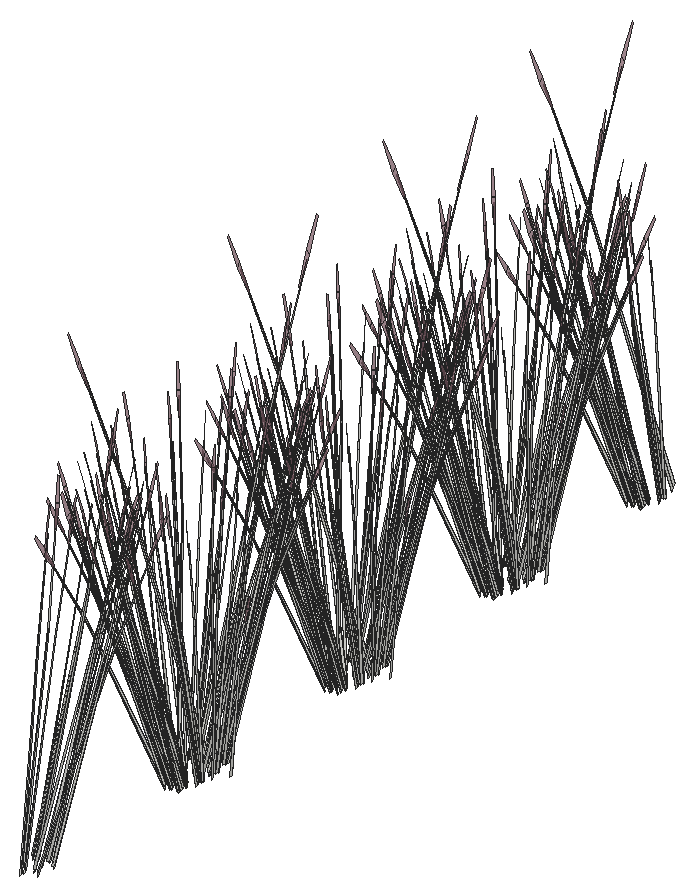
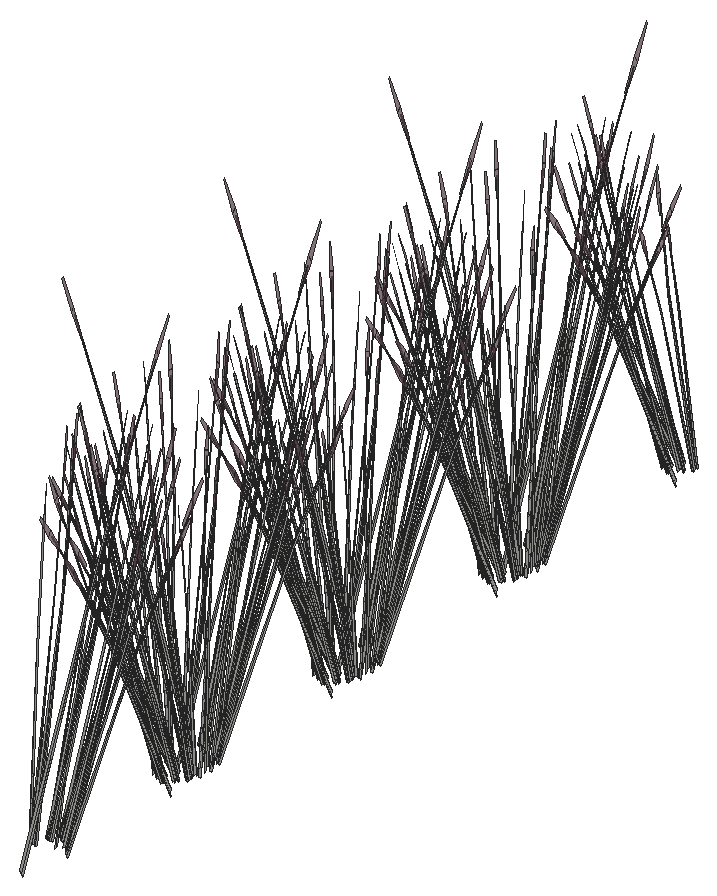
# SketchUp Ruby script. Lengths in inches.
U = 1.inch
M = Sketchup.active_model
def pt(a) = Geom::Point3d.new(a.map { |v| v * U })
def face(e, loops, mat)
  f = e.add_face(loops[0].map { |a| pt(a) })
  loops[1..].each { |l| e.add_face(l.map { |a| pt(a) }).erase! }
  f.material = f.back_material = mat if mat
  f
end
# faces: each face lists its corners as indices into pts; further lists are holes
def faces(e, pts, list, mat = nil) = list.each { |f| face(e, (f[0].is_a?(Array) ? f : [f]).map { |l| l.map { |i| pts[i] } }, mat) }
# xy, xz, yz: faces in a plane at the given z, y or x. An outline is a flat list of corners, or four numbers for a rectangle; further outlines are holes
def ring(l) = l.size == 4 ? [[l[0], l[1]], [l[2], l[1]], [l[2], l[3]], [l[0], l[3]]] : l.each_slice(2).to_a
def flat(e, list, mat, &to3) = list.each { |f| face(e, (f[0].is_a?(Array) ? f : [f]).map { |l| ring(l).map { |u, v| to3.(u, v) } }, mat) }
def xy(e, z, list, mat = nil) = flat(e, list, mat) { |x, y| [x, y, z] }
def xz(e, y, list, mat = nil) = flat(e, list, mat) { |x, z| [x, y, z] }
def yz(e, x, list, mat = nil) = flat(e, list, mat) { |y, z| [x, y, z] }
def lines(e, pts, list) = list.each { |a, b| e.add_line(pt(pts[a]), pt(pts[b])) }
# prism: a flat outline (further loops are holes) pulled along v
def prism(e, loops, v, mat = nil)
  f = face(e, loops, mat); d = Geom::Vector3d.new(v.map { |x| x * U })
  f.pushpull(f.normal.samedirection?(d) ? d.length : -d.length)
end
def box(e, o, s, mat = nil) = prism(e, [[o, [o[0] + s[0], o[1], o[2]], [o[0] + s[0], o[1] + s[1], o[2]], [o[0], o[1] + s[1], o[2]]]], [0, 0, s[2]], mat)
def at(x, y, z, deg = 0) = Geom::Transformation.translation(pt([x, y, z])) * Geom::Transformation.rotation(ORIGIN, Z_AXIS, deg.degrees)
def axes(o, x, y, z) = Geom::Transformation.new([*x, 0, *y, 0, *z, 0, *pt(o).to_a, 1])
def part(name) = M.definitions.add(name)
# library, detail: a bought-in or finely detailed component or shape, given as its bounding box
def library(name, o, s) = part(name).tap { |d| box(d.entities, o, s) }
def detail(e, o, s) = box(e.add_group.entities, o, s)
def put(e, d, t, mat = nil) = e.add_instance(d, t).tap { |i| i.material = mat if mat }
def group(e, t, mat = nil) = e.add_group.tap { |g| g.transformation = t; g.material = mat if mat }.entities
root = M.entities
M.materials.add("LightPink_Translucent").color = [144, 107, 117]
M.materials["LightPink_Translucent"].alpha = 0.75
c1 = part("blade")
p = [[2.15,0.21,22],[0,0.17,0],[0.09,0.45,0],[2.18,0.31,22],[2.29,0.31,22],[0.38,0.45,0],
  [2.48,0.24,33],[2.49,0.24,33],[2.48,0.22,33]]
faces(c1.entities,p,[[0,1,2,3],[4,5,2,3],[6,3,4,7],[8,0,3,6]])
c2 = part("seeds")
p = [[0.3,-0.1,1.38],[-0.01,-0.03,1.59],[-0.01,-0.03,0.03],[0.14,-0.07,-0.07],[0.29,-0.03,3],[0.15,0.01,3.11]]
faces(c2.entities,p,[[0,1,2,3],[1,0,4,5]],"LightPink_Translucent")
c3 = part("blade with seeds")
put(c3.entities,c1,at(0,0,0))
put(c3.entities,c2,axes([2.4,0.25,30.99],[1.5799,-0.05474,1.17369],[-0.12525,1.92788,0.29478],[-0.07173,-0.02425,1.56792]))
put(root,c3,axes([251.98,134.81,2.85],[0.15252,-0.52338,-0.08826],[0.22088,0.30152,-0.48986],[0.07678,0.14787,0.74434]))
put(root,c3,axes([250.875,132.91,2.01],[0.06393,-0.18788,1.24382],[0.16142,0.50711,0.10057],[-0.11071,0.23094,0.53172]))
put(root,c3,axes([250.67,133.46,2.59],[0.06575,0.55831,-0.37087],[-0.24901,0.09767,-0.28727],[-0.07136,0.14996,0.70962]))
put(root,c3,axes([252.16,134.55,2.59],[0.25257,-0.14535,-0.37087],[0.04418,0.55045,-0.28727],[0.06784,0.15774,0.70962]))
put(root,c3,axes([250.83,133.375,2.01],[0.04766,-0.21017,1.24382],[0.19993,0.43493,0.10057],[-0.09019,0.27107,0.53172]))
put(root,c3,axes([250.88,134.56,2.48],[-0.17318,0.32193,-0.25703],[-0.16394,-0.36759,0.33183],[-0.02494,0.18677,0.63492]))
put(root,c3,axes([251.38,134.83,2.85],[0.25047,-0.28468,-0.08826],[0.12309,0.50526,-0.48986],[0.03305,0.21292,0.74434]))
put(root,c3,axes([251.06,134.41,2.83],[0.18323,0.41084,-0.41166],[-0.19356,0.3598,-0.31887],[-0.02788,0.20874,0.78768]))
put(root,c3,axes([251.6,134.81,2.59],[0.25161,0.15328,-0.37087],[-0.08624,0.52553,-0.28727],[0.02307,0.21159,0.70962]))
put(root,c3,axes([251.74,133.72,2.01],[-0.05851,-0.19632,1.24382],[0.27036,-0.16528,0.10057],[0.0611,0.3082,0.53172]))
put(root,c3,axes([251.48,135.13,2.48],[-0.07716,0.47021,-0.25703],[-0.22512,-0.13715,0.33183],[0.02064,0.18932,0.63492]))
put(root,c3,axes([251,134.22,3.07],[-0.00666,0.56559,-0.57235],[-0.28045,-0.03799,0.06907],[-0.0296,0.23961,0.80965]))
put(root,c3,axes([251.26,133.82,2.01],[-0.00626,-0.23468,1.24382],[0.27152,0.15569,0.10057],[-0.01679,0.33444,0.53172]))
put(root,c3,axes([251.51,134.71,2.81],[0.12216,0.49718,-0.51563],[-0.25147,0.27708,0.06223],[0.02857,0.24022,0.72942]))
put(root,c3,axes([250.9,135.02,1.63],[0.00562,-0.31565,1.12021],[0.25293,0.16673,0.1548],[-0.02192,0.33641,0.52896]))
put(root,c3,axes([251.1,147.52,2.01],[0.05851,0.19632,1.24382],[-0.27036,0.16528,0.10057],[-0.0611,-0.3082,0.53172]))
put(root,c3,axes([251.82,147.67,2.81],[-0.12216,-0.49718,-0.51563],[0.25147,-0.27708,0.06223],[-0.02857,-0.24022,0.72942]))
put(root,c3,axes([252.33,148.15,2.81],[0.00666,-0.56559,-0.51563],[0.28045,0.03799,0.06223],[0.0296,-0.23961,0.72942]))
put(root,c3,axes([251.84,147.24,2.48],[0.07716,-0.47021,-0.25703],[0.22512,0.13715,0.33183],[-0.02064,-0.18932,0.63492]))
put(root,c3,axes([252.01,147.87,2.01],[-0.04766,0.21017,1.24382],[-0.19993,-0.43493,0.10057],[0.09019,-0.27107,0.53172]))
put(root,c3,axes([251.73,147.57,2.59],[-0.25161,-0.15328,-0.37087],[0.08624,-0.52553,-0.28727],[-0.02307,-0.21159,0.70962]))
put(root,c3,axes([252.27,147.97,2.59],[-0.18323,-0.41084,-0.37087],[0.19356,-0.3598,-0.28727],[0.02788,-0.20874,0.70962]))
put(root,c3,axes([251.94,147.54,2.85],[-0.25047,0.28468,-0.08826],[-0.12309,-0.50526,-0.48986],[-0.03305,-0.21292,0.74434]))
put(root,c3,axes([252.46,148.18,2.85],[-0.2813,-0.0303,-0.08826],[0.00769,-0.57361,-0.48986],[0.01954,-0.22092,0.74434]))
put(root,c3,axes([252.44,147.8125,2.48],[0.17318,-0.32193,-0.25703],[0.16394,0.36759,0.33183],[0.02494,-0.18677,0.63492]))
put(root,c3,axes([251.27,147.81,2.81],[-0.21825,-0.29555,-0.51563],[0.15511,-0.5179,0.06223],[-0.07907,-0.17646,0.72942]))
put(root,c3,axes([251.19,147.42,2.48],[-0.03953,-0.49251,-0.25703],[0.22598,-0.13005,0.33183],[-0.0607,-0.14114,0.63492]))
put(root,c3,axes([250.71,148.13,2.01],[0.09507,0.10535,1.24382],[-0.19675,0.44195,0.10057],[-0.12263,-0.19937,0.53172]))
put(root,c3,axes([251.17,147.82,2.59],[-0.25257,0.14535,-0.37087],[-0.04418,-0.55045,-0.28727],[-0.06784,-0.15774,0.70962]))
put(root,c3,axes([252.66,149.14,2.81],[0.1337,-0.48245,-0.51563],[0.23429,0.34287,0.06223],[0.07983,-0.1748,0.72942]))
put(root,c3,axes([252.65,148.91,2.59],[-0.06575,-0.55831,-0.37087],[0.24901,-0.09767,-0.28727],[0.07136,-0.14996,0.70962]))
put(root,c3,axes([252.77,149.31,2.85],[-0.23676,-0.33715,-0.08826],[0.1364,-0.48826,-0.48986],[0.06689,-0.16972,0.74434]))
put(root,c3,axes([251.79,151.15,1.61],[0.22119,0.24656,1.09782],[-0.21669,0.53118,0.43413],[-0.09706,-0.31482,0.92034]))
put(root,c3,axes([252.84,148.97,2.48],[0.2228,-0.08739,-0.25703],[0.05883,0.49954,0.33183],[0.06385,-0.13418,0.63492]))
put(root,c3,axes([250.67,148.28,2.48],[-0.14563,-0.38283,-0.25703],[0.16629,-0.3624,0.33183],[-0.08449,-0.05514,0.63492]))
put(root,c3,axes([250.82,148.54,2.81],[-0.25586,-0.01472,-0.51563],[0.01718,-0.61995,0.06223],[-0.1084,-0.06542,0.72942]))
put(root,c3,axes([250.74,148.66,2.59],[-0.18586,0.40503,-0.37087],[-0.16277,-0.42787,-0.28727],[-0.09443,-0.06163,0.70962]))
put(root,c3,axes([250.84,148.24,2.85],[-0.0137,0.62183,-0.08826],[-0.25949,-0.017,-0.48986],[-0.09994,-0.0432,0.74434]))
put(root,c3,axes([252.78,150.625,2.85],[-0.12878,-0.55367,-0.08826],[0.22857,-0.27208,-0.48986],[0.09632,-0.07305,0.74434]))
put(root,c3,axes([252.77,150.15,2.59],[0.06934,-0.55619,-0.37087],[0.23774,0.19064,-0.28727],[0.09572,-0.051,0.70962]))
put(root,c3,axes([250.51,149.1,2.01],[0.10617,-0.01385,1.24382],[-0.07043,0.60021,0.10057],[-0.1513,-0.03712,0.53172]))
put(root,c3,axes([252.72,150.35,2.81],[0.22491,-0.27005,-0.51563],[0.12534,0.55588,0.06223],[0.10867,-0.06315,0.72942]))
put(root,c3,axes([252.91,150.4,2.48],[0.21272,0.17057,-0.25703],[-0.06204,0.49764,0.33183],[0.08564,-0.04563,0.63492]))
put(root,c3,axes([250.41,149.61,2.48],[-0.21272,-0.17057,-0.25703],[0.06204,-0.49764,0.33183],[-0.08564,0.04563,0.63492]))
put(root,c3,axes([252.33,149.79,2.01],[-0.10617,0.01385,1.24382],[0.07043,-0.60021,0.10057],[0.1513,0.03712,0.53172]))
put(root,c3,axes([251.0625,149.53,1.62],[0.07276,-0.08845,1.2851],[0.02509,0.61759,0.10057],[-0.15759,0.08195,0.4593]))
put(root,c3,axes([250.56,149.87,2.59],[-0.06934,0.55619,-0.37087],[-0.23774,-0.19064,-0.28727],[-0.09572,0.051,0.70962]))
put(root,c3,axes([250.55,149.39,2.85],[0.12878,0.55367,-0.08826],[-0.22857,0.27208,-0.48986],[-0.09632,0.07305,0.74434]))
put(root,c3,axes([253.09,151.79,2.04],[-0.04899,-0.514,-0.02534],[0.23154,-0.11817,-0.1149],[0.04835,0.03259,0.37899]))
put(root,c3,axes([252.49,151.78,2.85],[0.0137,-0.62183,-0.08826],[0.25949,0.017,-0.48986],[0.09994,0.0432,0.74434]))
put(root,c3,axes([250.55,150.15,2.01],[0.08881,-0.12933,1.24382],[0.07477,0.59764,0.10057],[-0.13942,0.13507,0.53172]))
put(root,c3,axes([252.5,151.48,2.81],[0.25586,0.01472,-0.51563],[-0.01718,0.61995,0.06223],[0.1084,0.06542,0.72942]))
put(root,c3,axes([252.66,151.73,2.48],[0.14563,0.38283,-0.25703],[-0.16629,0.3624,0.33183],[0.08449,0.05514,0.63492]))
put(root,c3,axes([250.49,151.05,2.48],[-0.2228,0.08739,-0.25703],[-0.05883,-0.49954,0.33183],[-0.06385,0.13418,0.63492]))
put(root,c3,axes([252.13,150.75,2.01],[-0.09507,-0.10535,1.24382],[0.19675,-0.44195,0.10057],[0.12263,0.19937,0.53172]))
put(root,c3,axes([252.15,149.36,2.44],[-0.22117,-0.3177,1.00363],[0.23354,-0.49464,0.43304],[0.07136,0.29809,0.97011]))
put(root,c3,axes([250.56,150.71,2.85],[0.23676,0.33715,-0.08826],[-0.1364,0.48826,-0.48986],[-0.06689,0.16972,0.74434]))
put(root,c3,axes([251.98,152.45,2.85],[0.15252,-0.52338,-0.08826],[0.22088,0.30152,-0.48986],[0.07678,0.14787,0.74434]))
put(root,c3,axes([250.875,150.55,2.01],[0.06393,-0.18788,1.24382],[0.16142,0.50711,0.10057],[-0.11071,0.23094,0.53172]))
put(root,c3,axes([250.67,151.11,2.59],[0.06575,0.55831,-0.37087],[-0.24901,0.09767,-0.28727],[-0.07136,0.14996,0.70962]))
put(root,c3,axes([252.16,152.19,2.59],[0.25257,-0.14535,-0.37087],[0.04418,0.55045,-0.28727],[0.06784,0.15774,0.70962]))
put(root,c3,axes([250.83,151.02,2.01],[0.04766,-0.21017,1.24382],[0.19993,0.43493,0.10057],[-0.09019,0.27107,0.53172]))
put(root,c3,axes([250.88,152.2,2.48],[-0.17318,0.32193,-0.25703],[-0.16394,-0.36759,0.33183],[-0.02494,0.18677,0.63492]))
put(root,c3,axes([251.38,152.47,2.85],[0.25047,-0.28468,-0.08826],[0.12309,0.50526,-0.48986],[0.03305,0.21292,0.74434]))
put(root,c3,axes([251.06,152.05,2.83],[0.18323,0.41084,-0.41166],[-0.19356,0.3598,-0.31887],[-0.02788,0.20874,0.78768]))
put(root,c3,axes([251.6,152.45,2.59],[0.25161,0.15328,-0.37087],[-0.08624,0.52553,-0.28727],[0.02307,0.21159,0.70962]))
put(root,c3,axes([251.74,151.36,2.01],[-0.05851,-0.19632,1.24382],[0.27036,-0.16528,0.10057],[0.0611,0.3082,0.53172]))
put(root,c3,axes([251.48,152.77,2.48],[-0.07716,0.47021,-0.25703],[-0.22512,-0.13715,0.33183],[0.02064,0.18932,0.63492]))
put(root,c3,axes([251,151.86,3.07],[-0.00666,0.56559,-0.57235],[-0.28045,-0.03799,0.06907],[-0.0296,0.23961,0.80965]))
put(root,c3,axes([251.26,151.46,2.01],[-0.00626,-0.23468,1.24382],[0.27152,0.15569,0.10057],[-0.01679,0.33444,0.53172]))
put(root,c3,axes([251.51,152.35,2.81],[0.12216,0.49718,-0.51563],[-0.25147,0.27708,0.06223],[0.02857,0.24022,0.72942]))
put(root,c3,axes([250.9,152.66,1.63],[0.00562,-0.31565,1.12021],[0.25293,0.16673,0.1548],[-0.02192,0.33641,0.52896]))
put(root,c3,axes([251.1,163.79,2.01],[0.05851,0.19632,1.24382],[-0.27036,0.16528,0.10057],[-0.0611,-0.3082,0.53172]))
put(root,c3,axes([251.82,163.9375,2.81],[-0.12216,-0.49718,-0.51563],[0.25147,-0.27708,0.06223],[-0.02857,-0.24022,0.72942]))
put(root,c3,axes([252.33,164.42,2.81],[0.00666,-0.56559,-0.51563],[0.28045,0.03799,0.06223],[0.0296,-0.23961,0.72942]))
put(root,c3,axes([251.84,163.51,2.48],[0.07716,-0.47021,-0.25703],[0.22512,0.13715,0.33183],[-0.02064,-0.18932,0.63492]))
put(root,c3,axes([252.01,164.14,2.01],[-0.04766,0.21017,1.24382],[-0.19993,-0.43493,0.10057],[0.09019,-0.27107,0.53172]))
put(root,c3,axes([251.73,163.84,2.59],[-0.25161,-0.15328,-0.37087],[0.08624,-0.52553,-0.28727],[-0.02307,-0.21159,0.70962]))
put(root,c3,axes([252.27,164.23,2.59],[-0.18323,-0.41084,-0.37087],[0.19356,-0.3598,-0.28727],[0.02788,-0.20874,0.70962]))
put(root,c3,axes([251.94,163.8125,2.85],[-0.25047,0.28468,-0.08826],[-0.12309,-0.50526,-0.48986],[-0.03305,-0.21292,0.74434]))
put(root,c3,axes([252.46,164.45,2.85],[-0.2813,-0.0303,-0.08826],[0.00769,-0.57361,-0.48986],[0.01954,-0.22092,0.74434]))
put(root,c3,axes([252.44,164.08,2.48],[0.17318,-0.32193,-0.25703],[0.16394,0.36759,0.33183],[0.02494,-0.18677,0.63492]))
put(root,c3,axes([251.27,164.08,2.81],[-0.21825,-0.29555,-0.51563],[0.15511,-0.5179,0.06223],[-0.07907,-0.17646,0.72942]))
put(root,c3,axes([251.19,163.6875,2.48],[-0.03953,-0.49251,-0.25703],[0.22598,-0.13005,0.33183],[-0.0607,-0.14114,0.63492]))
put(root,c3,axes([250.71,164.4,2.01],[0.09507,0.10535,1.24382],[-0.19675,0.44195,0.10057],[-0.12263,-0.19937,0.53172]))
put(root,c3,axes([251.17,164.09,2.59],[-0.25257,0.14535,-0.37087],[-0.04418,-0.55045,-0.28727],[-0.06784,-0.15774,0.70962]))
put(root,c3,axes([252.66,165.41,2.81],[0.1337,-0.48245,-0.51563],[0.23429,0.34287,0.06223],[0.07983,-0.1748,0.72942]))
put(root,c3,axes([252.65,165.18,2.59],[-0.06575,-0.55831,-0.37087],[0.24901,-0.09767,-0.28727],[0.07136,-0.14996,0.70962]))
put(root,c3,axes([252.77,165.58,2.85],[-0.23676,-0.33715,-0.08826],[0.1364,-0.48826,-0.48986],[0.06689,-0.16972,0.74434]))
put(root,c3,axes([251.79,167.42,1.61],[0.22119,0.24656,1.09782],[-0.21669,0.53118,0.43413],[-0.09706,-0.31482,0.92034]))
put(root,c3,axes([252.84,165.24,2.48],[0.2228,-0.08739,-0.25703],[0.05883,0.49954,0.33183],[0.06385,-0.13418,0.63492]))
put(root,c3,axes([250.67,164.55,2.48],[-0.14563,-0.38283,-0.25703],[0.16629,-0.3624,0.33183],[-0.08449,-0.05514,0.63492]))
put(root,c3,axes([250.82,164.81,2.81],[-0.25586,-0.01472,-0.51563],[0.01718,-0.61995,0.06223],[-0.1084,-0.06542,0.72942]))
put(root,c3,axes([250.74,164.93,2.59],[-0.18586,0.40503,-0.37087],[-0.16277,-0.42787,-0.28727],[-0.09443,-0.06163,0.70962]))
put(root,c3,axes([250.84,164.51,2.85],[-0.0137,0.62183,-0.08826],[-0.25949,-0.017,-0.48986],[-0.09994,-0.0432,0.74434]))
put(root,c3,axes([252.78,166.9,2.85],[-0.12878,-0.55367,-0.08826],[0.22857,-0.27208,-0.48986],[0.09632,-0.07305,0.74434]))
put(root,c3,axes([252.77,166.42,2.59],[0.06934,-0.55619,-0.37087],[0.23774,0.19064,-0.28727],[0.09572,-0.051,0.70962]))
put(root,c3,axes([250.51,165.37,2.01],[0.10617,-0.01385,1.24382],[-0.07043,0.60021,0.10057],[-0.1513,-0.03712,0.53172]))
put(root,c3,axes([252.72,166.62,2.81],[0.22491,-0.27005,-0.51563],[0.12534,0.55588,0.06223],[0.10867,-0.06315,0.72942]))
put(root,c3,axes([252.91,166.67,2.48],[0.21272,0.17057,-0.25703],[-0.06204,0.49764,0.33183],[0.08564,-0.04563,0.63492]))
put(root,c3,axes([250.41,165.88,2.48],[-0.21272,-0.17057,-0.25703],[0.06204,-0.49764,0.33183],[-0.08564,0.04563,0.63492]))
put(root,c3,axes([252.33,166.06,2.01],[-0.10617,0.01385,1.24382],[0.07043,-0.60021,0.10057],[0.1513,0.03712,0.53172]))
put(root,c3,axes([251.0625,165.8,1.62],[0.07276,-0.08845,1.2851],[0.02509,0.61759,0.10057],[-0.15759,0.08195,0.4593]))
put(root,c3,axes([250.56,166.13,2.59],[-0.06934,0.55619,-0.37087],[-0.23774,-0.19064,-0.28727],[-0.09572,0.051,0.70962]))
put(root,c3,axes([250.55,165.66,2.85],[0.12878,0.55367,-0.08826],[-0.22857,0.27208,-0.48986],[-0.09632,0.07305,0.74434]))
put(root,c3,axes([253.09,168.0625,2.04],[-0.04899,-0.514,-0.02534],[0.23154,-0.11817,-0.1149],[0.04835,0.03259,0.37899]))
put(root,c3,axes([252.49,168.05,2.85],[0.0137,-0.62183,-0.08826],[0.25949,0.017,-0.48986],[0.09994,0.0432,0.74434]))
put(root,c3,axes([250.55,166.42,2.01],[0.08881,-0.12933,1.24382],[0.07477,0.59764,0.10057],[-0.13942,0.13507,0.53172]))
put(root,c3,axes([252.5,167.75,2.81],[0.25586,0.01472,-0.51563],[-0.01718,0.61995,0.06223],[0.1084,0.06542,0.72942]))
put(root,c3,axes([252.66,168,2.48],[0.14563,0.38283,-0.25703],[-0.16629,0.3624,0.33183],[0.08449,0.05514,0.63492]))
put(root,c3,axes([250.49,167.32,2.48],[-0.2228,0.08739,-0.25703],[-0.05883,-0.49954,0.33183],[-0.06385,0.13418,0.63492]))
put(root,c3,axes([252.13,167.02,2.01],[-0.09507,-0.10535,1.24382],[0.19675,-0.44195,0.10057],[0.12263,0.19937,0.53172]))
put(root,c3,axes([252.15,165.63,2.44],[-0.22117,-0.3177,1.00363],[0.23354,-0.49464,0.43304],[0.07136,0.29809,0.97011]))
put(root,c3,axes([250.56,166.98,2.85],[0.23676,0.33715,-0.08826],[-0.1364,0.48826,-0.48986],[-0.06689,0.16972,0.74434]))
put(root,c3,axes([251.98,168.72,2.85],[0.15252,-0.52338,-0.08826],[0.22088,0.30152,-0.48986],[0.07678,0.14787,0.74434]))
put(root,c3,axes([250.875,166.82,2.01],[0.06393,-0.18788,1.24382],[0.16142,0.50711,0.10057],[-0.11071,0.23094,0.53172]))
put(root,c3,axes([250.67,167.375,2.59],[0.06575,0.55831,-0.37087],[-0.24901,0.09767,-0.28727],[-0.07136,0.14996,0.70962]))
put(root,c3,axes([252.16,168.46,2.59],[0.25257,-0.14535,-0.37087],[0.04418,0.55045,-0.28727],[0.06784,0.15774,0.70962]))
put(root,c3,axes([250.83,167.29,2.01],[0.04766,-0.21017,1.24382],[0.19993,0.43493,0.10057],[-0.09019,0.27107,0.53172]))
put(root,c3,axes([250.88,168.47,2.48],[-0.17318,0.32193,-0.25703],[-0.16394,-0.36759,0.33183],[-0.02494,0.18677,0.63492]))
put(root,c3,axes([251.38,168.74,2.85],[0.25047,-0.28468,-0.08826],[0.12309,0.50526,-0.48986],[0.03305,0.21292,0.74434]))
put(root,c3,axes([251.06,168.32,2.83],[0.18323,0.41084,-0.41166],[-0.19356,0.3598,-0.31887],[-0.02788,0.20874,0.78768]))
put(root,c3,axes([251.6,168.72,2.59],[0.25161,0.15328,-0.37087],[-0.08624,0.52553,-0.28727],[0.02307,0.21159,0.70962]))
put(root,c3,axes([251.74,167.63,2.01],[-0.05851,-0.19632,1.24382],[0.27036,-0.16528,0.10057],[0.0611,0.3082,0.53172]))
put(root,c3,axes([251.48,169.04,2.48],[-0.07716,0.47021,-0.25703],[-0.22512,-0.13715,0.33183],[0.02064,0.18932,0.63492]))
put(root,c3,axes([251,168.13,3.07],[-0.00666,0.56559,-0.57235],[-0.28045,-0.03799,0.06907],[-0.0296,0.23961,0.80965]))
put(root,c3,axes([251.26,167.73,2.01],[-0.00626,-0.23468,1.24382],[0.27152,0.15569,0.10057],[-0.01679,0.33444,0.53172]))
put(root,c3,axes([251.51,168.62,2.81],[0.12216,0.49718,-0.51563],[-0.25147,0.27708,0.06223],[0.02857,0.24022,0.72942]))
put(root,c3,axes([251.1,179.64,2.01],[0.05851,0.19632,1.24382],[-0.27036,0.16528,0.10057],[-0.0611,-0.3082,0.53172]))
put(root,c3,axes([250.9,168.93,1.63],[0.00562,-0.31565,1.12021],[0.25293,0.16673,0.1548],[-0.02192,0.33641,0.52896]))
put(root,c3,axes([251.82,179.79,2.81],[-0.12216,-0.49718,-0.51563],[0.25147,-0.27708,0.06223],[-0.02857,-0.24022,0.72942]))
put(root,c3,axes([252.33,180.27,2.81],[0.00666,-0.56559,-0.51563],[0.28045,0.03799,0.06223],[0.0296,-0.23961,0.72942]))
put(root,c3,axes([251.84,179.37,2.48],[0.07716,-0.47021,-0.25703],[0.22512,0.13715,0.33183],[-0.02064,-0.18932,0.63492]))
put(root,c3,axes([252.01,179.99,2.01],[-0.04766,0.21017,1.24382],[-0.19993,-0.43493,0.10057],[0.09019,-0.27107,0.53172]))
put(root,c3,axes([251.73,179.6875,2.59],[-0.25161,-0.15328,-0.37087],[0.08624,-0.52553,-0.28727],[-0.02307,-0.21159,0.70962]))
put(root,c3,axes([252.27,180.09,2.59],[-0.18323,-0.41084,-0.37087],[0.19356,-0.3598,-0.28727],[0.02788,-0.20874,0.70962]))
put(root,c3,axes([251.94,179.66,2.85],[-0.25047,0.28468,-0.08826],[-0.12309,-0.50526,-0.48986],[-0.03305,-0.21292,0.74434]))
put(root,c3,axes([252.46,180.3,2.85],[-0.2813,-0.0303,-0.08826],[0.00769,-0.57361,-0.48986],[0.01954,-0.22092,0.74434]))
put(root,c3,axes([252.44,179.93,2.48],[0.17318,-0.32193,-0.25703],[0.16394,0.36759,0.33183],[0.02494,-0.18677,0.63492]))
put(root,c3,axes([251.27,179.93,2.81],[-0.21825,-0.29555,-0.51563],[0.15511,-0.5179,0.06223],[-0.07907,-0.17646,0.72942]))
put(root,c3,axes([251.19,179.54,2.48],[-0.03953,-0.49251,-0.25703],[0.22598,-0.13005,0.33183],[-0.0607,-0.14114,0.63492]))
put(root,c3,axes([250.71,180.25,2.01],[0.09507,0.10535,1.24382],[-0.19675,0.44195,0.10057],[-0.12263,-0.19937,0.53172]))
put(root,c3,axes([251.17,179.94,2.59],[-0.25257,0.14535,-0.37087],[-0.04418,-0.55045,-0.28727],[-0.06784,-0.15774,0.70962]))
put(root,c3,axes([252.66,181.26,2.81],[0.1337,-0.48245,-0.51563],[0.23429,0.34287,0.06223],[0.07983,-0.1748,0.72942]))
put(root,c3,axes([252.65,181.03,2.59],[-0.06575,-0.55831,-0.37087],[0.24901,-0.09767,-0.28727],[0.07136,-0.14996,0.70962]))
put(root,c3,axes([252.77,181.43,2.85],[-0.23676,-0.33715,-0.08826],[0.1364,-0.48826,-0.48986],[0.06689,-0.16972,0.74434]))
put(root,c3,axes([251.79,183.27,1.61],[0.22119,0.24656,1.09782],[-0.21669,0.53118,0.43413],[-0.09706,-0.31482,0.92034]))
put(root,c3,axes([252.84,181.09,2.48],[0.2228,-0.08739,-0.25703],[0.05883,0.49954,0.33183],[0.06385,-0.13418,0.63492]))
put(root,c3,axes([250.67,180.4,2.48],[-0.14563,-0.38283,-0.25703],[0.16629,-0.3624,0.33183],[-0.08449,-0.05514,0.63492]))
put(root,c3,axes([250.82,180.66,2.81],[-0.25586,-0.01472,-0.51563],[0.01718,-0.61995,0.06223],[-0.1084,-0.06542,0.72942]))
put(root,c3,axes([250.74,180.78,2.59],[-0.18586,0.40503,-0.37087],[-0.16277,-0.42787,-0.28727],[-0.09443,-0.06163,0.70962]))
put(root,c3,axes([250.84,180.36,2.85],[-0.0137,0.62183,-0.08826],[-0.25949,-0.017,-0.48986],[-0.09994,-0.0432,0.74434]))
put(root,c3,axes([252.78,182.75,2.85],[-0.12878,-0.55367,-0.08826],[0.22857,-0.27208,-0.48986],[0.09632,-0.07305,0.74434]))
put(root,c3,axes([252.77,182.27,2.59],[0.06934,-0.55619,-0.37087],[0.23774,0.19064,-0.28727],[0.09572,-0.051,0.70962]))
put(root,c3,axes([250.51,181.22,2.01],[0.10617,-0.01385,1.24382],[-0.07043,0.60021,0.10057],[-0.1513,-0.03712,0.53172]))
put(root,c3,axes([252.72,182.47,2.81],[0.22491,-0.27005,-0.51563],[0.12534,0.55588,0.06223],[0.10867,-0.06315,0.72942]))
put(root,c3,axes([252.91,182.53,2.48],[0.21272,0.17057,-0.25703],[-0.06204,0.49764,0.33183],[0.08564,-0.04563,0.63492]))
put(root,c3,axes([250.41,181.73,2.48],[-0.21272,-0.17057,-0.25703],[0.06204,-0.49764,0.33183],[-0.08564,0.04563,0.63492]))
put(root,c3,axes([252.33,181.91,2.01],[-0.10617,0.01385,1.24382],[0.07043,-0.60021,0.10057],[0.1513,0.03712,0.53172]))
put(root,c3,axes([251.0625,181.65,1.62],[0.07276,-0.08845,1.2851],[0.02509,0.61759,0.10057],[-0.15759,0.08195,0.4593]))
put(root,c3,axes([250.56,181.99,2.59],[-0.06934,0.55619,-0.37087],[-0.23774,-0.19064,-0.28727],[-0.09572,0.051,0.70962]))
put(root,c3,axes([250.55,181.51,2.85],[0.12878,0.55367,-0.08826],[-0.22857,0.27208,-0.48986],[-0.09632,0.07305,0.74434]))
put(root,c3,axes([253.09,183.91,2.04],[-0.04899,-0.514,-0.02534],[0.23154,-0.11817,-0.1149],[0.04835,0.03259,0.37899]))
put(root,c3,axes([252.49,183.9,2.85],[0.0137,-0.62183,-0.08826],[0.25949,0.017,-0.48986],[0.09994,0.0432,0.74434]))
put(root,c3,axes([250.55,182.27,2.01],[0.08881,-0.12933,1.24382],[0.07477,0.59764,0.10057],[-0.13942,0.13507,0.53172]))
put(root,c3,axes([252.5,183.6,2.81],[0.25586,0.01472,-0.51563],[-0.01718,0.61995,0.06223],[0.1084,0.06542,0.72942]))
put(root,c3,axes([252.66,183.85,2.48],[0.14563,0.38283,-0.25703],[-0.16629,0.3624,0.33183],[0.08449,0.05514,0.63492]))
put(root,c3,axes([250.49,183.17,2.48],[-0.2228,0.08739,-0.25703],[-0.05883,-0.49954,0.33183],[-0.06385,0.13418,0.63492]))
put(root,c3,axes([252.13,182.87,2.01],[-0.09507,-0.10535,1.24382],[0.19675,-0.44195,0.10057],[0.12263,0.19937,0.53172]))
put(root,c3,axes([252.15,181.49,2.44],[-0.22117,-0.3177,1.00363],[0.23354,-0.49464,0.43304],[0.07136,0.29809,0.97011]))
put(root,c3,axes([250.56,182.83,2.85],[0.23676,0.33715,-0.08826],[-0.1364,0.48826,-0.48986],[-0.06689,0.16972,0.74434]))
put(root,c3,axes([251.98,184.57,2.85],[0.15252,-0.52338,-0.08826],[0.22088,0.30152,-0.48986],[0.07678,0.14787,0.74434]))
put(root,c3,axes([250.875,182.68,2.01],[0.06393,-0.18788,1.24382],[0.16142,0.50711,0.10057],[-0.11071,0.23094,0.53172]))
put(root,c3,axes([250.67,183.23,2.59],[0.06575,0.55831,-0.37087],[-0.24901,0.09767,-0.28727],[-0.07136,0.14996,0.70962]))
put(root,c3,axes([252.16,184.3125,2.59],[0.25257,-0.14535,-0.37087],[0.04418,0.55045,-0.28727],[0.06784,0.15774,0.70962]))
put(root,c3,axes([250.83,183.14,2.01],[0.04766,-0.21017,1.24382],[0.19993,0.43493,0.10057],[-0.09019,0.27107,0.53172]))
put(root,c3,axes([250.88,184.32,2.48],[-0.17318,0.32193,-0.25703],[-0.16394,-0.36759,0.33183],[-0.02494,0.18677,0.63492]))
put(root,c3,axes([251.38,184.6,2.85],[0.25047,-0.28468,-0.08826],[0.12309,0.50526,-0.48986],[0.03305,0.21292,0.74434]))
put(root,c3,axes([251.06,184.17,2.83],[0.18323,0.41084,-0.41166],[-0.19356,0.3598,-0.31887],[-0.02788,0.20874,0.78768]))
put(root,c3,axes([251.6,184.57,2.59],[0.25161,0.15328,-0.37087],[-0.08624,0.52553,-0.28727],[0.02307,0.21159,0.70962]))
put(root,c3,axes([251.74,183.49,2.01],[-0.05851,-0.19632,1.24382],[0.27036,-0.16528,0.10057],[0.0611,0.3082,0.53172]))
put(root,c3,axes([251.48,184.89,2.48],[-0.07716,0.47021,-0.25703],[-0.22512,-0.13715,0.33183],[0.02064,0.18932,0.63492]))
put(root,c3,axes([251,183.98,3.07],[-0.00666,0.56559,-0.57235],[-0.28045,-0.03799,0.06907],[-0.0296,0.23961,0.80965]))
put(root,c3,axes([251.26,183.58,2.01],[-0.00626,-0.23468,1.24382],[0.27152,0.15569,0.10057],[-0.01679,0.33444,0.53172]))
put(root,c3,axes([251.1,194.63,2.01],[0.05851,0.19632,1.24382],[-0.27036,0.16528,0.10057],[-0.0611,-0.3082,0.53172]))
put(root,c3,axes([251.51,184.47,2.81],[0.12216,0.49718,-0.51563],[-0.25147,0.27708,0.06223],[0.02857,0.24022,0.72942]))
put(root,c3,axes([251.82,194.77,2.81],[-0.12216,-0.49718,-0.51563],[0.25147,-0.27708,0.06223],[-0.02857,-0.24022,0.72942]))
put(root,c3,axes([252.33,195.26,2.81],[0.00666,-0.56559,-0.51563],[0.28045,0.03799,0.06223],[0.0296,-0.23961,0.72942]))
put(root,c3,axes([251.84,194.35,2.48],[0.07716,-0.47021,-0.25703],[0.22512,0.13715,0.33183],[-0.02064,-0.18932,0.63492]))
put(root,c3,axes([252.01,194.97,2.01],[-0.04766,0.21017,1.24382],[-0.19993,-0.43493,0.10057],[0.09019,-0.27107,0.53172]))
put(root,c3,axes([250.9,184.78,1.63],[0.00562,-0.31565,1.12021],[0.25293,0.16673,0.1548],[-0.02192,0.33641,0.52896]))
put(root,c3,axes([251.73,194.67,2.59],[-0.25161,-0.15328,-0.37087],[0.08624,-0.52553,-0.28727],[-0.02307,-0.21159,0.70962]))
put(root,c3,axes([252.27,195.07,2.59],[-0.18323,-0.41084,-0.37087],[0.19356,-0.3598,-0.28727],[0.02788,-0.20874,0.70962]))
put(root,c3,axes([251.94,194.65,2.85],[-0.25047,0.28468,-0.08826],[-0.12309,-0.50526,-0.48986],[-0.03305,-0.21292,0.74434]))
put(root,c3,axes([252.46,195.29,2.85],[-0.2813,-0.0303,-0.08826],[0.00769,-0.57361,-0.48986],[0.01954,-0.22092,0.74434]))
put(root,c3,axes([252.44,194.92,2.48],[0.17318,-0.32193,-0.25703],[0.16394,0.36759,0.33183],[0.02494,-0.18677,0.63492]))
put(root,c3,axes([251.27,194.91,2.81],[-0.21825,-0.29555,-0.51563],[0.15511,-0.5179,0.06223],[-0.07907,-0.17646,0.72942]))
put(root,c3,axes([251.19,194.52,2.48],[-0.03953,-0.49251,-0.25703],[0.22598,-0.13005,0.33183],[-0.0607,-0.14114,0.63492]))
put(root,c3,axes([250.71,195.24,2.01],[0.09507,0.10535,1.24382],[-0.19675,0.44195,0.10057],[-0.12263,-0.19937,0.53172]))
put(root,c3,axes([251.17,194.93,2.59],[-0.25257,0.14535,-0.37087],[-0.04418,-0.55045,-0.28727],[-0.06784,-0.15774,0.70962]))
put(root,c3,axes([252.66,196.24,2.81],[0.1337,-0.48245,-0.51563],[0.23429,0.34287,0.06223],[0.07983,-0.1748,0.72942]))
put(root,c3,axes([252.65,196.02,2.59],[-0.06575,-0.55831,-0.37087],[0.24901,-0.09767,-0.28727],[0.07136,-0.14996,0.70962]))
put(root,c3,axes([252.77,196.42,2.85],[-0.23676,-0.33715,-0.08826],[0.1364,-0.48826,-0.48986],[0.06689,-0.16972,0.74434]))
put(root,c3,axes([251.79,198.26,1.61],[0.22119,0.24656,1.09782],[-0.21669,0.53118,0.43413],[-0.09706,-0.31482,0.92034]))
put(root,c3,axes([252.84,196.08,2.48],[0.2228,-0.08739,-0.25703],[0.05883,0.49954,0.33183],[0.06385,-0.13418,0.63492]))
put(root,c3,axes([250.67,195.39,2.48],[-0.14563,-0.38283,-0.25703],[0.16629,-0.3624,0.33183],[-0.08449,-0.05514,0.63492]))
put(root,c3,axes([250.82,195.65,2.81],[-0.25586,-0.01472,-0.51563],[0.01718,-0.61995,0.06223],[-0.1084,-0.06542,0.72942]))
